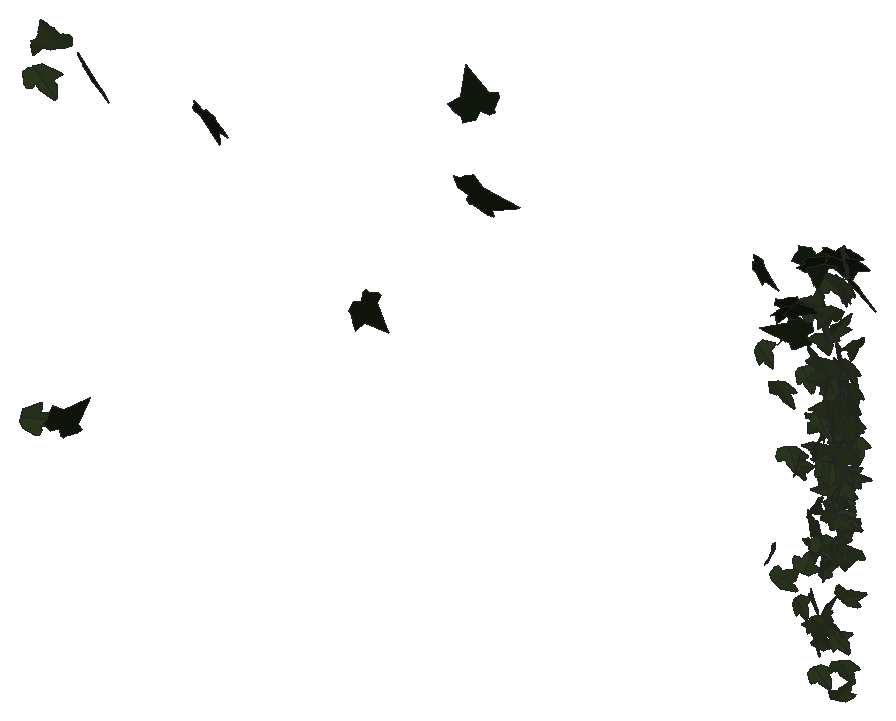
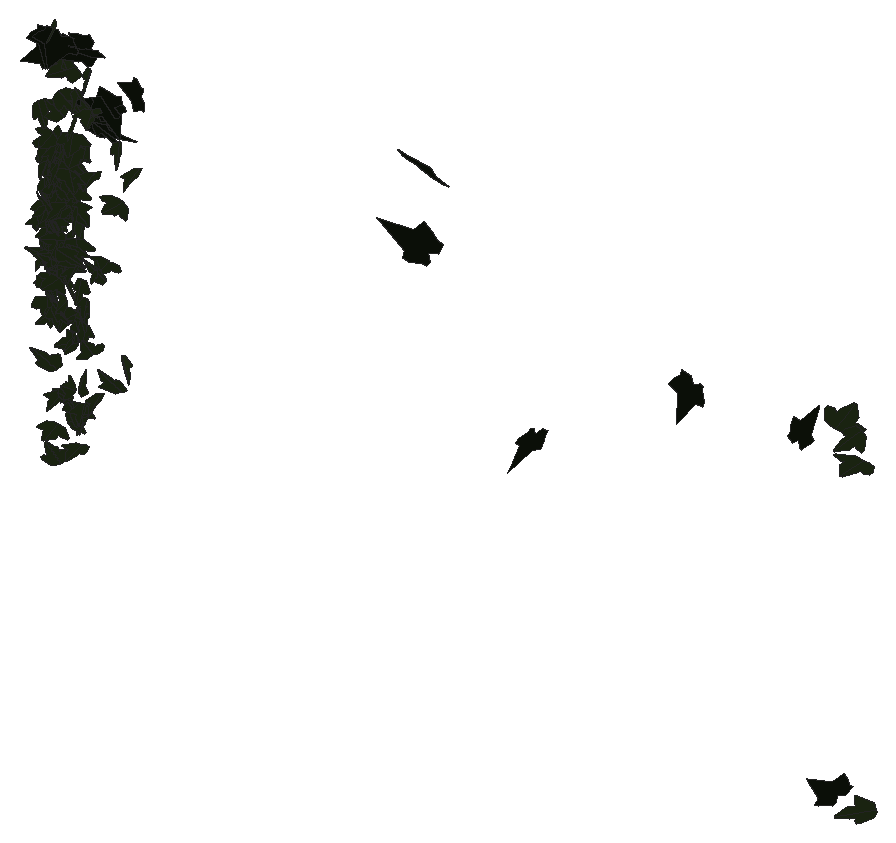
# SketchUp Ruby script. Lengths in inches.
U = 1.inch
M = Sketchup.active_model
def pt(a) = Geom::Point3d.new(a.map { |v| v * U })
def face(e, loops, mat)
  f = e.add_face(loops[0].map { |a| pt(a) })
  loops[1..].each { |l| e.add_face(l.map { |a| pt(a) }).erase! }
  f.material = f.back_material = mat if mat
  f
end
# faces: each face lists its corners as indices into pts; further lists are holes
def faces(e, pts, list, mat = nil) = list.each { |f| face(e, (f[0].is_a?(Array) ? f : [f]).map { |l| l.map { |i| pts[i] } }, mat) }
# xy, xz, yz: faces in a plane at the given z, y or x. An outline is a flat list of corners, or four numbers for a rectangle; further outlines are holes
def ring(l) = l.size == 4 ? [[l[0], l[1]], [l[2], l[1]], [l[2], l[3]], [l[0], l[3]]] : l.each_slice(2).to_a
def flat(e, list, mat, &to3) = list.each { |f| face(e, (f[0].is_a?(Array) ? f : [f]).map { |l| ring(l).map { |u, v| to3.(u, v) } }, mat) }
def xy(e, z, list, mat = nil) = flat(e, list, mat) { |x, y| [x, y, z] }
def xz(e, y, list, mat = nil) = flat(e, list, mat) { |x, z| [x, y, z] }
def yz(e, x, list, mat = nil) = flat(e, list, mat) { |y, z| [x, y, z] }
def lines(e, pts, list) = list.each { |a, b| e.add_line(pt(pts[a]), pt(pts[b])) }
# prism: a flat outline (further loops are holes) pulled along v
def prism(e, loops, v, mat = nil)
  f = face(e, loops, mat); d = Geom::Vector3d.new(v.map { |x| x * U })
  f.pushpull(f.normal.samedirection?(d) ? d.length : -d.length)
end
def box(e, o, s, mat = nil) = prism(e, [[o, [o[0] + s[0], o[1], o[2]], [o[0] + s[0], o[1] + s[1], o[2]], [o[0], o[1] + s[1], o[2]]]], [0, 0, s[2]], mat)
def at(x, y, z, deg = 0) = Geom::Transformation.translation(pt([x, y, z])) * Geom::Transformation.rotation(ORIGIN, Z_AXIS, deg.degrees)
def axes(o, x, y, z) = Geom::Transformation.new([*x, 0, *y, 0, *z, 0, *pt(o).to_a, 1])
def part(name) = M.definitions.add(name)
# library, detail: a bought-in or finely detailed component or shape, given as its bounding box
def library(name, o, s) = part(name).tap { |d| box(d.entities, o, s) }
def detail(e, o, s) = box(e.add_group.entities, o, s)
def put(e, d, t, mat = nil) = e.add_instance(d, t).tap { |i| i.material = mat if mat }
def group(e, t, mat = nil) = e.add_group.tap { |g| g.transformation = t; g.material = mat if mat }.entities
root = M.entities
M.materials.add("1026 AP 7946 SUNNY SIDE UP").color = [254, 231, 186]
M.materials.add("efeu1").color = [18, 25, 13]
M.materials.add("efeu2").color = [43, 57, 29]
c1 = part("ivyleaf_10")
p = [[0,0.5,-0.03],[-0.0625,2.02,-0.43],[-0.19,2.01,-0.46],[-0.54,1.05,-0.29],[-0.52,0.625,-0.18],[-0.83,0.76,-0.28],
  [-1.16,0.64,-0.33],[-1.15,0.33,-0.24],[-0.77,-0.39,0.02],[-0.3,-0.51,0.16],[0.04,-0.48,0.23],[-0.02,2.01,-0.4375],
  [-0.06,2.01,-0.43],[0.04,-0.49,0.23],[0.67,-0.49,0.14],[1.38,0.36,-0.2],[1.375,0.51,-0.24],[0.81,0.65,-0.19],
  [0.62,0.59,-0.15],[0.6,1.09,-0.28],[0.5,1.23,-0.31]]
faces(c1.entities,p,[[0,1,2,3,4,5,6,7,8,9,10],[11,12,0,13,14,15,16,17,18,19,20]],"efeu2")
c2 = part("ivyleaf_9")
p = [[1.54,2.16,1.25],[1.36,2.04,1.19],[-0.21,0.99,0.68],[-0.71,1.11,0.82],[-0.85,0.86,0.67],[-0.8,0.17,0.21],
  [-0.9,-0.01,0.1],[-0.67,-0.16,-0.02],[-0.08,-0.08,-0.05],[-0.03,-0.6,-0.4],[0.65,-0.88,-0.66],[0.83,-0.6,-0.49],
  [1.29,-0.42,-0.43],[1.8125,-0.07,-0.26],[1.21,0.44,0.15]]
faces(c2.entities,p,[[0,1,2,3,4,5,6,7,8,9,10,11,12,13,14]],"efeu1")
put(root,c1,axes([122.8,213.09,255.66],[0.00835,0.05286,0.29831],[0.16526,0.26986,-0.05122],[-0.43183,0.10429,-0.01383]),"1026 AP 7946 SUNNY SIDE UP")
put(root,c1,axes([122.94,213.29,265.23],[-0.09984,-0.12765,-0.24766],[0.19722,0.20452,-0.14525],[0.3787,-0.14016,0.01035]),"1026 AP 7946 SUNNY SIDE UP")
put(root,c1,axes([122.97,213.15,264.44],[0.29893,0.14075,0.15331],[0.21063,0.06673,-0.24223],[-0.24246,0.23151,-0.02142]),"1026 AP 7946 SUNNY SIDE UP")
put(root,c1,axes([123.4375,213.25,265.33],[-0.36144,-0.09542,-0.13441],[-0.20374,-0.02524,0.25512],[-0.15079,0.26283,-0.02254]),"1026 AP 7946 SUNNY SIDE UP")
put(root,c2,axes([123.68,213.09,255.75],[-0.10021,-0.01801,0.29865],[0.37076,0.17028,0.06528],[-0.26696,0.24324,-0.02145]),"1026 AP 7946 SUNNY SIDE UP")
put(root,c2,axes([124.53,213.32,264.59],[0.20512,-0.23952,0.12946],[-0.06225,0.12263,0.28081],[-0.42174,-0.1346,0.02152]),"1026 AP 7946 SUNNY SIDE UP")
put(root,c2,axes([127.51,213.4,264.91],[0.41973,-0.04342,-0.16303],[-0.25124,-0.00196,-0.27754],[0.05717,0.31019,-0.02272]),"1026 AP 7946 SUNNY SIDE UP")
put(root,c2,axes([132.21,213.11,261.87],[0.10693,-0.15676,-0.29176],[-0.19151,0.25476,-0.17445],[0.47026,0.13939,-0.0047]),"1026 AP 7946 SUNNY SIDE UP")
put(root,c2,axes([135.3,213.37,267.76],[-0.49924,0.0749,-0.10491],[-0.14359,0.0561,0.33477],[0.13822,0.32881,-0.03114]),"1026 AP 7946 SUNNY SIDE UP")
put(root,c2,axes([135.15,213.27,265.59],[0.14933,-0.04691,0.3344],[0.40627,-0.19789,-0.10841],[0.31831,0.27458,-0.01851]),"1026 AP 7946 SUNNY SIDE UP")
put(root,c1,axes([143.45,213.18,264.62],[0.01272,0.2201,0.0912],[0.01341,0.087,-0.22633],[-0.37206,0.01066,-0.00504]),"1026 AP 7946 SUNNY SIDE UP")
put(root,c2,axes([143.26,213.25,266.67],[0.10434,-0.04259,-0.24209],[0.37344,-0.01149,0.07124],[-0.03585,-0.24368,0.03748]),"1026 AP 7946 SUNNY SIDE UP")
put(root,c1,axes([143.78,213.37,265.23],[-0.22243,0.14486,0.11316],[-0.13162,0.07047,-0.20795],[-0.25288,-0.1641,0.0087]),"1026 AP 7946 SUNNY SIDE UP")
put(root,c1,axes([143.81,213.1,259.66],[0.06854,-0.2075,-0.07973],[-0.03871,0.07264,-0.21782],[0.34542,0.04931,-0.00859]),"1026 AP 7946 SUNNY SIDE UP")
put(root,c1,axes([143.83,213.32,263.75],[-0.29165,0.02259,-0.13386],[0.19001,-0.06126,-0.18885],[-0.08358,-0.2181,0.03778]),"1026 AP 7946 SUNNY SIDE UP")
put(root,c1,axes([143.98,213.16,258.97],[0.25769,-0.01994,-0.14678],[0.22504,0.0023,0.16941],[-0.0213,-0.21707,0.014]),"1026 AP 7946 SUNNY SIDE UP")
put(root,c2,axes([144.31,213.07,266.03],[-0.00028,0.23733,-0.08298],[0.00316,-0.08189,-0.24497],[-0.39476,-0.00083,-0.0019]),"1026 AP 7946 SUNNY SIDE UP")
put(root,c1,axes([144.1,213.34,262.17],[0.29776,0.06217,0.08746],[0.13488,0.00875,-0.20453],[-0.09504,0.20719,-0.01628]),"1026 AP 7946 SUNNY SIDE UP")
put(root,c2,axes([144.59,213.23,265.37],[-0.27328,0.04029,0.17076],[-0.2646,-0.00376,-0.1811],[-0.04174,-0.23998,0.03006]),"1026 AP 7946 SUNNY SIDE UP")
put(root,c1,axes([144.31,213.51,262],[-0.02153,0.12445,-0.17469],[-0.03494,-0.17054,-0.12756],[-0.32979,0.00995,0.02492]),"1026 AP 7946 SUNNY SIDE UP")
put(root,c2,axes([144.51,213.16,265.65],[-0.18428,0.17982,-0.12397],[0.08983,-0.10748,-0.22154],[-0.32908,-0.13004,0.00895]),"1026 AP 7946 SUNNY SIDE UP")
put(root,c1,axes([144.21,213.46,261.84],[0.11004,-0.06238,-0.19537],[0.25402,-0.09974,0.0948],[-0.18354,-0.17544,0.01408]),"1026 AP 7946 SUNNY SIDE UP")
put(root,c1,axes([144.45,213.6,266.92],[-0.17496,0.20832,0.0305],[-0.04232,0.01778,-0.24269],[-0.32788,-0.11346,0.01505]),"1026 AP 7946 SUNNY SIDE UP")
put(root,c2,axes([144.18,213.07,265.97],[0.18895,0.03593,0.21395],[0.32511,0.02505,-0.12769],[-0.06262,0.23845,-0.01738]),"1026 AP 7946 SUNNY SIDE UP")
put(root,c1,axes([144.42,213.52,265.96],[0.16158,0.20376,0.01944],[0.00403,0.01854,-0.23491],[-0.32158,0.10262,0.00682]),"1026 AP 7946 SUNNY SIDE UP")
put(root,c1,axes([144.49,213.1875,258.56],[0.01747,0.20289,0.07126],[0.00081,0.06808,-0.2089],[-0.33647,0.0107,0.00319]),"1026 AP 7946 SUNNY SIDE UP")
put(root,c1,axes([144.49,213.41,264.3],[0.11886,0.20805,0.04117],[0.04042,0.03185,-0.22745],[-0.33031,0.07876,-0.01302]),"1026 AP 7946 SUNNY SIDE UP")
put(root,c1,axes([144.89,213.375,266.11],[-0.0379,0.06901,0.23761],[-0.35222,0.07749,-0.04763],[-0.1371,-0.21816,0.05668]),"1026 AP 7946 SUNNY SIDE UP")
put(root,c1,axes([144.74,213.36,264.9],[-0.2659,0.15488,-0.02308],[0.01053,-0.02709,-0.23586],[-0.24604,-0.16854,0.01485]),"1026 AP 7946 SUNNY SIDE UP")
put(root,c1,axes([144.84,213.52,262.48],[-0.27403,-0.104,0.03383],[-0.03475,-0.02807,-0.20884],[0.16822,-0.17522,0.01196]),"1026 AP 7946 SUNNY SIDE UP")
put(root,c1,axes([144.88,213.21,260.63],[-0.22221,0.10842,0.10675],[-0.14342,0.04982,-0.18265],[-0.18635,-0.16763,0.01329]),"1026 AP 7946 SUNNY SIDE UP")
put(root,c1,axes([144.74,213.08,259.57],[0.1625,0.15652,-0.13112],[0.09746,0.1125,0.19368],[0.30279,-0.1202,0.00803]),"1026 AP 7946 SUNNY SIDE UP")
put(root,c1,axes([144.86,213.19,260.82],[-0.23371,0.13866,0.04292],[-0.05989,0.01898,-0.20893],[-0.21927,-0.15297,0.01133]),"1026 AP 7946 SUNNY SIDE UP")
put(root,c1,axes([144.79,213.62,266.23],[-0.16742,0.2,-0.04944],[0.00117,-0.05492,-0.23237],[-0.32383,-0.1036,0.02472]),"1026 AP 7946 SUNNY SIDE UP")
put(root,c1,axes([144.9,213.7,264.29],[-0.33306,0.02561,0.04184],[-0.07255,-0.05999,-0.21004],[-0.02017,-0.20713,0.06467]),"1026 AP 7946 SUNNY SIDE UP")
put(root,c1,axes([144.83,213.65,265.57],[-0.09866,0.21796,-0.00631],[-0.00466,-0.00851,-0.23365],[-0.34289,-0.0626,0.00499]),"1026 AP 7946 SUNNY SIDE UP")
put(root,c1,axes([144.85,213.64,265.22],[-0.24369,-0.15787,-0.03366],[0.0692,0.00091,-0.22573],[0.24357,-0.1582,0.03045]),"1026 AP 7946 SUNNY SIDE UP")
put(root,c1,axes([144.93,213.17,260.18],[-0.30056,0.06146,0.03264],[-0.05496,-0.0067,-0.20615],[-0.09352,-0.19358,0.01625]),"1026 AP 7946 SUNNY SIDE UP")
put(root,c2,axes([144.8,213.41,267.37],[-0.20996,-0.17966,-0.09615],[0.14274,0.04548,-0.22619],[0.28372,-0.15583,0.04264]),"1026 AP 7946 SUNNY SIDE UP")
put(root,c1,axes([144.88,213.23,258.1875],[0.06094,0.20264,0.04706],[-0.05346,0.05089,-0.20779],[-0.32182,0.02992,0.04343]),"1026 AP 7946 SUNNY SIDE UP")
put(root,c1,axes([145.06,213.38,263.27],[-0.24177,-0.09341,0.13557],[-0.15548,-0.09004,-0.18465],[0.2014,-0.18164,0.0202]),"1026 AP 7946 SUNNY SIDE UP")
put(root,c1,axes([144.91,213.6,262.38],[0.31553,-0.0182,-0.03437],[-0.05395,-0.01095,-0.20715],[0.02536,0.20311,-0.01304]),"1026 AP 7946 SUNNY SIDE UP")
put(root,c1,axes([145.08,213.7,262.25],[0.18422,-0.00433,-0.17362],[-0.26504,-0.00141,-0.1207],[0.00206,0.20523,-0.00329]),"1026 AP 7946 SUNNY SIDE UP")
put(root,c1,axes([145.01,213.33,263.1],[-0.10346,0.14323,0.1648],[-0.15282,0.12839,-0.15966],[-0.3,-0.1148,0.02449]),"1026 AP 7946 SUNNY SIDE UP")
put(root,c1,axes([144.96,213.18,258.62],[-0.21567,0.16583,0.00488],[0.01816,0.00464,0.22139],[0.26019,0.13713,-0.01141]),"1026 AP 7946 SUNNY SIDE UP")
put(root,c1,axes([144.9,213.25,257.84],[-0.15103,0.17607,-0.05131],[0.02194,-0.05017,-0.20658],[-0.28731,-0.09639,0.0112]),"1026 AP 7946 SUNNY SIDE UP")
put(root,c1,axes([145.18,213.27,264.39],[-0.15691,0.03277,0.20684],[-0.31712,0.01175,-0.10527],[-0.03964,-0.22373,0.02343]),"1026 AP 7946 SUNNY SIDE UP")
put(root,c2,axes([144.78,213.14,267.27],[0.22498,0.11038,0.16885],[0.20449,0.09872,-0.18559],[-0.23285,0.19335,0.00016]),"1026 AP 7946 SUNNY SIDE UP")
put(root,c1,axes([144.92,213.31,262.61],[-0.00625,-0.09626,-0.20838],[0.00099,-0.20177,0.09799],[-0.35146,0.00114,0.00398]),"1026 AP 7946 SUNNY SIDE UP")
put(root,c1,axes([145.02,213.21,258.12],[-0.33068,-0.02108,0.00196],[0.00004,-0.02049,-0.21684],[0.03329,-0.20931,0.01978]),"1026 AP 7946 SUNNY SIDE UP")
put(root,c1,axes([145.1875,213.21,257.74],[-0.20786,0.04491,-0.1566],[-0.20869,0.07745,0.14269],[0.13695,0.18617,-0.02024]),"1026 AP 7946 SUNNY SIDE UP")
put(root,c1,axes([145.01,213.15,261.23],[-0.03286,-0.17308,-0.13212],[0.02965,0.12589,-0.17884],[0.33649,-0.028,0.00286]),"1026 AP 7946 SUNNY SIDE UP")
put(root,c1,axes([144.99,213.66,263.4375],[0.06706,0.16569,-0.1323],[-0.05376,-0.12478,-0.17697],[-0.32613,0.05464,0.00196]),"1026 AP 7946 SUNNY SIDE UP")
put(root,c1,axes([145.125,213.15,260.39],[-0.06511,0.07482,-0.20568],[-0.10804,0.1883,0.08829],[0.31803,0.07929,-0.01212]),"1026 AP 7946 SUNNY SIDE UP")
put(root,c1,axes([144.95,213.49,261.79],[0.03066,0.20434,0.00913],[0.01005,0.00713,-0.21134],[-0.32137,0.01972,-0.00574]),"1026 AP 7946 SUNNY SIDE UP")
put(root,c1,axes([145.01,213.4,264.75],[-0.34484,-0.03968,-0.03179],[0.05263,-0.01357,-0.22883],[0.05868,-0.22102,0.01842]),"1026 AP 7946 SUNNY SIDE UP")
put(root,c1,axes([145.01,213.73,263.39],[0.07284,0.12271,0.17068],[0.08093,0.15681,-0.13413],[-0.31302,0.0691,0.00504]),"1026 AP 7946 SUNNY SIDE UP")
put(root,c1,axes([145.24,213.47,266.0625],[-0.13899,-0.17882,0.13199],[-0.06805,-0.12235,-0.20578],[0.34009,-0.09756,0.01277]),"1026 AP 7946 SUNNY SIDE UP")
put(root,c1,axes([145.2,213.22,263.5625],[-0.26327,-0.15082,-0.01947],[0.03833,-0.00017,-0.23154],[0.23575,-0.1684,0.0159]),"1026 AP 7946 SUNNY SIDE UP")
put(root,c1,axes([145.41,213.56,260.66],[-0.03358,0.05313,0.20098],[-0.30248,0.05413,-0.03662],[-0.09642,-0.18833,0.04489]),"1026 AP 7946 SUNNY SIDE UP")
put(root,c1,axes([145.2,213.24,258.53],[0.0532,-0.12043,0.16587],[-0.06112,0.15698,0.12975],[-0.31108,-0.05144,0.00287]),"1026 AP 7946 SUNNY SIDE UP")
put(root,c1,axes([145.09,213.1,257.05],[0.13761,0.16335,0.09864],[0.07826,0.08087,-0.19037],[-0.28649,0.10055,-0.00462]),"1026 AP 7946 SUNNY SIDE UP")
put(root,c1,axes([145.26,213.43,260.77],[0.04569,0.00022,0.20989],[-0.11945,0.19097,0.01206],[-0.29725,-0.0767,0.02742]),"1026 AP 7946 SUNNY SIDE UP")
put(root,c1,axes([145.14,213.09,263.55],[0.09618,0.2115,0.04585],[0.02697,0.04011,-0.22652],[-0.33839,0.06331,-0.00502]),"1026 AP 7946 SUNNY SIDE UP")
put(root,c1,axes([145.43,213.39,261.7],[0.09564,0.00801,-0.2148],[-0.29862,-0.08796,-0.06106],[-0.13609,0.19864,-0.01698]),"1026 AP 7946 SUNNY SIDE UP")
put(root,c1,axes([145.2,213.23,259.8125],[0.00497,0.16881,-0.11678],[0.00121,-0.11434,-0.17458],[-0.32057,0.00219,-0.00247]),"1026 AP 7946 SUNNY SIDE UP")
put(root,c1,axes([145.18,213.63,263.99],[0.34068,-0.00036,0.02623],[0.03981,-0.02056,-0.22234],[0.00433,0.21718,-0.01973]),"1026 AP 7946 SUNNY SIDE UP")
put(root,c1,axes([145.3,213.18,263.83],[-0.21543,-0.17083,-0.0016],[0.01847,-0.00868,-0.22514],[0.26797,-0.13673,0.01423]),"1026 AP 7946 SUNNY SIDE UP")
put(root,c1,axes([145.24,213.15,259.66],[0.02934,-0.04626,0.21284],[0.00464,0.2077,0.04879],[-0.33327,-0.00118,0.01941]),"1026 AP 7946 SUNNY SIDE UP")
put(root,c1,axes([145.28,213.71,262.35],[-0.09578,0.18827,-0.05721],[-0.02297,-0.06343,-0.20152],[-0.30827,-0.05377,0.03279]),"1026 AP 7946 SUNNY SIDE UP")
put(root,c1,axes([145.3,213.57,264.42],[0.29245,-0.12478,-0.02611],[-0.03381,0.01216,-0.23065],[0.19711,0.18722,-0.00083]),"1026 AP 7946 SUNNY SIDE UP")
put(root,c1,axes([145.23,213.17,262.26],[0.1239,0.19956,0.00607],[0.01368,0.00168,-0.22088],[-0.31357,0.07892,-0.00724]),"1026 AP 7946 SUNNY SIDE UP")
put(root,c1,axes([145.28,213.56,263.69],[-0.31541,-0.08614,-0.04932],[0.09303,-0.01979,-0.22109],[0.12346,-0.20516,0.04061]),"1026 AP 7946 SUNNY SIDE UP")
put(root,c1,axes([145.07,213.45,266.8125],[0.22971,0.01973,0.19389],[0.25289,0.11209,-0.14014],[-0.15646,0.21014,0.05814]),"1026 AP 7946 SUNNY SIDE UP")
put(root,c2,axes([145.26,213.55,267.56],[0.29699,0.14256,-0.05431],[-0.04089,-0.05382,-0.24255],[-0.23591,0.18879,-0.02632]),"1026 AP 7946 SUNNY SIDE UP")
put(root,c1,axes([145.32,213.53,263.33],[-0.3132,0.0825,-0.04255],[0.03349,-0.05559,-0.21809],[-0.14149,-0.19578,0.04255]),"1026 AP 7946 SUNNY SIDE UP")
put(root,c1,axes([145.45,213.15,261.21],[0.17925,-0.15392,-0.1361],[-0.1374,0.09838,-0.1965],[0.28684,0.14331,-0.00907]),"1026 AP 7946 SUNNY SIDE UP")
put(root,c1,axes([145.27,213.55,264.71],[-0.17152,0.17353,-0.10127],[0.06169,-0.09233,-0.21118],[-0.30825,-0.11503,0.01409]),"1026 AP 7946 SUNNY SIDE UP")
put(root,c1,axes([145.37,213.57,264.24],[-0.10373,0.18126,0.113],[-0.06776,0.0999,-0.19805],[-0.32533,-0.0786,0.00522]),"1026 AP 7946 SUNNY SIDE UP")
put(root,c1,axes([145.33,213.54,265.09],[-0.16821,0.2025,-0.0337],[-0.00716,-0.04051,-0.23501],[-0.32275,-0.10464,0.02278]),"1026 AP 7946 SUNNY SIDE UP")
put(root,c1,axes([145.35,213.24,264.4],[0.03517,0.17764,-0.13309],[-0.06253,-0.12546,-0.18412],[-0.34062,0.04137,0.02006]),"1026 AP 7946 SUNNY SIDE UP")
put(root,c1,axes([145.28,213.65,263.8],[0.29877,-0.08751,0.05827],[0.07062,-0.03851,-0.21513],[0.14831,0.19462,-0.01495]),"1026 AP 7946 SUNNY SIDE UP")
put(root,c1,axes([145.33,213.57,263.99],[-0.12166,0.20038,-0.0394],[0.00597,-0.0407,-0.22123],[-0.32105,-0.07669,0.01082]),"1026 AP 7946 SUNNY SIDE UP")
put(root,c1,axes([145.19,213.125,260.39],[0.26203,0.06005,0.12794],[0.19153,0.02622,-0.18179],[-0.10078,0.20597,-0.01283]),"1026 AP 7946 SUNNY SIDE UP")
put(root,c1,axes([145.33,213.53,262.41],[0.01252,-0.07971,0.20551],[0.02774,0.19965,0.08244],[-0.33732,0.01346,0.01441]),"1026 AP 7946 SUNNY SIDE UP")
put(root,c1,axes([145.34,213.47,265.61],[-0.03817,-0.1953,0.13135],[0.01349,0.12847,0.2034],[-0.36745,0.025,-0.00617]),"1026 AP 7946 SUNNY SIDE UP")
put(root,c1,axes([145.48,213.08,263.65],[0.08233,-0.01847,-0.22789],[-0.06343,0.2226,-0.02769],[0.34307,0.04559,0.04957]),"1026 AP 7946 SUNNY SIDE UP")
put(root,c1,axes([145.35,213.29,263.28],[0.1906,0.17607,-0.007],[0.008,-0.01295,-0.21997],[-0.27701,0.12077,-0.01117]),"1026 AP 7946 SUNNY SIDE UP")
put(root,c1,axes([145.41,213.62,263.63],[-0.09575,0.17407,0.12169],[0.07427,-0.10746,0.18918],[0.32143,0.07668,-0.00746]),"1026 AP 7946 SUNNY SIDE UP")
put(root,c1,axes([145.39,213.61,262.87],[0.2334,0.14356,-0.03902],[-0.03205,-0.03451,-0.21266],[-0.23158,0.14946,-0.0099]),"1026 AP 7946 SUNNY SIDE UP")
put(root,c1,axes([145.37,213.58,262.79],[0.09736,-0.20569,-0.02657],[0.0193,-0.02201,0.22109],[-0.32516,-0.06289,0.00517]),"1026 AP 7946 SUNNY SIDE UP")
put(root,c1,axes([145.41,213.16,262.3],[0.09575,0.19445,-0.06318],[-0.03121,-0.05921,-0.21026],[-0.31961,0.06403,0.0016]),"1026 AP 7946 SUNNY SIDE UP")
put(root,c1,axes([145.45,213.63,262.97],[0.11954,-0.19471,0.04631],[0.01919,-0.04467,-0.21555],[0.31403,0.07685,-0.00446]),"1026 AP 7946 SUNNY SIDE UP")
put(root,c1,axes([145.41,213.56,264.73],[0.02886,0.22229,-0.01627],[0.00125,-0.01717,-0.22987],[-0.35055,0.01824,-0.00216]),"1026 AP 7946 SUNNY SIDE UP")
put(root,c1,axes([145.35,213.64,261.43],[-0.26751,0.00851,-0.11262],[0.16364,-0.05129,-0.17119],[-0.05453,-0.19564,0.03875]),"1026 AP 7946 SUNNY SIDE UP")
put(root,c1,axes([145.53,213.08,260.31],[-0.06472,0.1083,0.18667],[-0.1313,0.16052,-0.11784],[-0.30395,-0.0924,0.01116]),"1026 AP 7946 SUNNY SIDE UP")
put(root,c1,axes([145.41,213.57,262.22],[-0.1025,0.18713,-0.06964],[0.03038,-0.06597,-0.2045],[-0.31194,-0.06791,0.00296]),"1026 AP 7946 SUNNY SIDE UP")
put(root,c1,axes([145.61,213.11,263.1],[0.16152,0.02182,0.19939],[-0.23986,0.14488,0.06747],[-0.19012,-0.16424,0.08428]),"1026 AP 7946 SUNNY SIDE UP")
put(root,c1,axes([145.48,213.23,261.58],[0.05757,-0.13778,0.15506],[-0.05697,0.1469,0.14771],[-0.31668,-0.05147,0.00162]),"1026 AP 7946 SUNNY SIDE UP")
put(root,c1,axes([145.46,213.6,263.0625],[-0.09124,0.20803,-0.0107],[-0.00341,-0.01261,-0.22249],[-0.32759,-0.05781,0.0053]),"1026 AP 7946 SUNNY SIDE UP")
put(root,c1,axes([145.48,213.125,263.31],[-0.14395,0.19584,-0.01103],[-0.00368,-0.01413,-0.22264],[-0.30848,-0.09122,0.0078]),"1026 AP 7946 SUNNY SIDE UP")
put(root,c1,axes([145.26,213.24,258.26],[0.00733,-0.00543,0.21093],[0.31385,-0.04599,-0.0062],[0.07251,0.19961,0.00554]),"1026 AP 7946 SUNNY SIDE UP")
put(root,c1,axes([145.55,213.39,266.93],[-0.33672,0.10249,0.0168],[-0.04337,-0.02152,-0.24257],[-0.15717,-0.21364,0.03094]),"1026 AP 7946 SUNNY SIDE UP")
put(root,c1,axes([145.38,213.54,261.92],[0.10155,0.06479,-0.19282],[0.1759,0.15099,0.09431],[0.25766,-0.12861,0.01161]),"1026 AP 7946 SUNNY SIDE UP")
put(root,c1,axes([145.47,213.39,261.49],[0.18059,0.16825,-0.04047],[-0.019,-0.04038,-0.2097],[-0.27136,0.1148,-0.01225]),"1026 AP 7946 SUNNY SIDE UP")
put(root,c1,axes([145.77,213.2,261.64],[-0.03287,0.02563,0.21143],[-0.31325,0.0524,-0.02736],[-0.08655,-0.19938,0.01872]),"1026 AP 7946 SUNNY SIDE UP")
put(root,c2,axes([145.53,213.45,267.46],[0.28598,0.15128,-0.0778],[-0.06498,-0.06906,-0.24271],[-0.25843,0.18478,-0.02506]),"1026 AP 7946 SUNNY SIDE UP")
put(root,c1,axes([145.625,213.14,260.3],[-0.30389,-0.07461,0.0179],[-0.01452,-0.02528,-0.21256],[0.11974,-0.19243,0.01966]),"1026 AP 7946 SUNNY SIDE UP")
put(root,c1,axes([145.66,213.15,262.25],[0.19907,-0.14128,-0.10052],[-0.10751,0.06863,-0.19498],[0.24687,0.14382,-0.00386]),"1026 AP 7946 SUNNY SIDE UP")
put(root,c1,axes([145.55,213.45,267.65],[-0.1178,0.23341,-0.04053],[0.00166,-0.04232,-0.2525],[-0.37254,-0.074,0.01169]),"1026 AP 7946 SUNNY SIDE UP")
put(root,c1,axes([145.58,213.64,263.24],[-0.24443,-0.1377,-0.05127],[0.09111,0.00758,-0.21136],[0.21097,-0.16281,0.03188]),"1026 AP 7946 SUNNY SIDE UP")
put(root,c1,axes([145.62,213.63,262.58],[0.00225,0.19975,0.06124],[-0.07593,0.05704,-0.19974],[-0.31826,-0.01219,0.04808]),"1026 AP 7946 SUNNY SIDE UP")
put(root,c1,axes([145.625,213.66,261.8125],[0.1585,-0.17567,0.02149],[0.00571,-0.0231,-0.20861],[0.27829,0.10052,-0.00796]),"1026 AP 7946 SUNNY SIDE UP")
put(root,c1,axes([145.64,213.36,261.875],[0.01287,0.15755,-0.13],[-0.06177,-0.12353,-0.1611],[-0.31222,0.03094,0.02651]),"1026 AP 7946 SUNNY SIDE UP")
put(root,c1,axes([145.78,213.28,261.97],[-0.2523,0.09288,0.10056],[-0.17495,-0.00709,-0.1825],[-0.11843,-0.1874,0.05537]),"1026 AP 7946 SUNNY SIDE UP")
put(root,c1,axes([145.625,213.64,262],[0.01198,0.17388,0.11116],[-0.01917,0.10719,-0.17806],[-0.32038,0.00009,0.01481]),"1026 AP 7946 SUNNY SIDE UP")
put(root,c1,axes([145.76,213.2,261.97],[0.27986,-0.01983,-0.11429],[-0.17627,-0.01193,-0.18333],[0.01646,0.20933,-0.02004]),"1026 AP 7946 SUNNY SIDE UP")
put(root,c1,axes([145.64,213.63,263.17],[0.04396,0.20705,-0.03905],[-0.03885,-0.03593,-0.21452],[-0.32903,0.0319,0.02012]),"1026 AP 7946 SUNNY SIDE UP")
put(root,c1,axes([145.63,213.36,262.73],[-0.22502,-0.12486,-0.08954],[0.11547,0.0467,-0.195],[0.20878,-0.16041,0.01134]),"1026 AP 7946 SUNNY SIDE UP")
put(root,c1,axes([145.72,213.18,262.81],[-0.3142,-0.08152,0.01196],[-0.00708,-0.0208,-0.22171],[0.12939,-0.1991,0.0169]),"1026 AP 7946 SUNNY SIDE UP")
put(root,c1,axes([145.63,213.22,261.74],[-0.05944,0.15298,-0.13316],[0.01608,-0.13077,-0.1622],[-0.31538,-0.0355,0.01682]),"1026 AP 7946 SUNNY SIDE UP")
put(root,c1,axes([145.68,213.67,263.36],[0.26117,-0.1343,0.00453],[-0.00965,-0.01578,-0.21952],[0.21111,0.16543,-0.01564]),"1026 AP 7946 SUNNY SIDE UP")
put(root,c1,axes([145.72,213.22,262.39],[0.22707,-0.16049,-0.02144],[-0.03849,0.00468,-0.22185],[0.25136,0.1457,-0.0146]),"1026 AP 7946 SUNNY SIDE UP")
put(root,c1,axes([145.66,213.18,256.59],[-0.14033,-0.17005,0.0717],[0.04114,0.06591,0.1981],[-0.28655,0.09274,-0.00667]),"1026 AP 7946 SUNNY SIDE UP")
put(root,c1,axes([145.49,213.61,261.92],[-0.08497,-0.03443,0.20336],[0.27836,0.08801,0.06618],[-0.14825,0.18498,0.00772]),"1026 AP 7946 SUNNY SIDE UP")
put(root,c1,axes([145.77,213.15,267],[-0.24664,0.1812,0.05606],[-0.07412,0.02965,-0.24618],[-0.28763,-0.16302,0.01537]),"1026 AP 7946 SUNNY SIDE UP")
put(root,c1,axes([145.84,213.26,261.04],[0.17773,-0.06561,-0.16245],[-0.1473,0.13379,-0.12604],[0.22392,0.14009,0.04603]),"1026 AP 7946 SUNNY SIDE UP")
put(root,c1,axes([145.58,213.35,260.58],[-0.01438,-0.09026,-0.19081],[0.1775,-0.15672,0.07222],[-0.27015,-0.09817,0.05761]),"1026 AP 7946 SUNNY SIDE UP")
put(root,c1,axes([145.72,213.33,264.02],[-0.01367,-0.21221,-0.07283],[0.08169,0.06571,-0.21304],[0.34148,-0.02422,0.04805]),"1026 AP 7946 SUNNY SIDE UP")
put(root,c1,axes([145.79,213.19,263.5625],[-0.2374,-0.1637,-0.00522],[0.01894,-0.00549,-0.22908],[0.25678,-0.15094,0.01207]),"1026 AP 7946 SUNNY SIDE UP")
put(root,c1,axes([145.6875,213.41,264.875],[-0.28072,0.09609,-0.09717],[0.10456,-0.07431,-0.20689],[-0.18479,-0.18802,0.03055]),"1026 AP 7946 SUNNY SIDE UP")
put(root,c1,axes([145.7,213.21,257.39],[-0.27243,-0.08047,-0.0827],[0.14531,-0.01588,-0.19026],[0.10319,-0.1901,0.04958]),"1026 AP 7946 SUNNY SIDE UP")
put(root,c1,axes([145.69,213.04,258.14],[0.08439,0.17592,0.11107],[0.03445,0.10488,-0.18867],[-0.32178,0.05736,0.00893]),"1026 AP 7946 SUNNY SIDE UP")
put(root,c1,axes([145.86,213.25,261.12],[-0.24154,-0.12229,0.05143],[-0.04776,-0.0429,-0.202],[0.20256,-0.15595,0.01369]),"1026 AP 7946 SUNNY SIDE UP")
put(root,c1,axes([145.6875,213.33,259.04],[-0.20088,-0.03778,0.16564],[0.22695,0.07382,0.13627],[-0.12691,0.19181,-0.01849]),"1026 AP 7946 SUNNY SIDE UP")
put(root,c1,axes([145.82,213.59,262.875],[0.06063,0.21137,-0.02414],[-0.00004,-0.02503,-0.22144],[-0.3346,0.0383,-0.00435]),"1026 AP 7946 SUNNY SIDE UP")
put(root,c1,axes([145.7,213.15,261.17],[-0.12944,-0.10973,-0.15774],[0.26611,0.02897,-0.11542],[0.12825,-0.17085,0.0803]),"1026 AP 7946 SUNNY SIDE UP")
put(root,c1,axes([145.93,213.44,265.54],[-0.05931,-0.23077,0.01514],[0.00427,-0.01666,-0.24093],[0.36371,-0.03743,0.0053]),"1026 AP 7946 SUNNY SIDE UP")
put(root,c2,axes([145.67,213.49,267.04],[0.31855,-0.13305,0.03396],[0.02154,-0.04021,-0.2485],[0.21474,0.2014,-0.02545]),"1026 AP 7946 SUNNY SIDE UP")
put(root,c1,axes([145.9,213.27,264.48],[-0.3086,0.10852,-0.03331],[0.02749,-0.03611,-0.23004],[-0.1762,-0.1957,0.02244]),"1026 AP 7946 SUNNY SIDE UP")
put(root,c1,axes([145.94,213.32,263.23],[0.1612,-0.19296,-0.00617],[-0.01822,-0.00062,-0.22484],[0.30296,0.10263,-0.01024]),"1026 AP 7946 SUNNY SIDE UP")
put(root,c1,axes([145.99,213.14,260.43],[-0.31866,-0.05109,0.0319],[-0.03947,-0.02767,-0.21444],[0.0855,-0.20318,0.0199]),"1026 AP 7946 SUNNY SIDE UP")
put(root,c1,axes([145.92,213.29,264.1],[-0.24739,0.15855,-0.0157],[0.00069,-0.02225,-0.2297],[-0.25058,-0.15659,0.01487]),"1026 AP 7946 SUNNY SIDE UP")
put(root,c1,axes([145.88,213.11,260.16],[-0.0198,-0.04633,-0.20545],[0.11051,0.18641,-0.04815],[0.30195,-0.07126,0.00415]),"1026 AP 7946 SUNNY SIDE UP")
